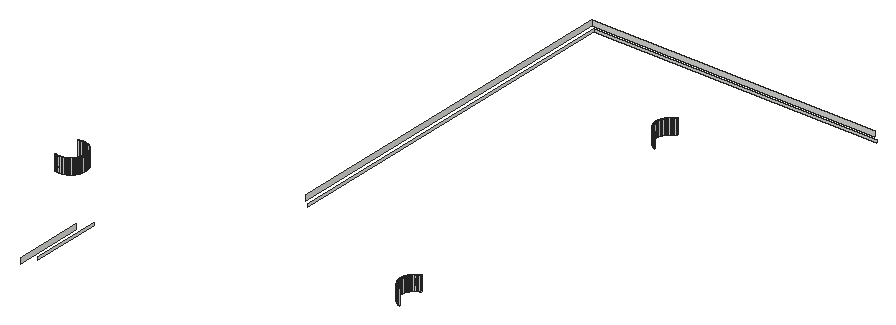
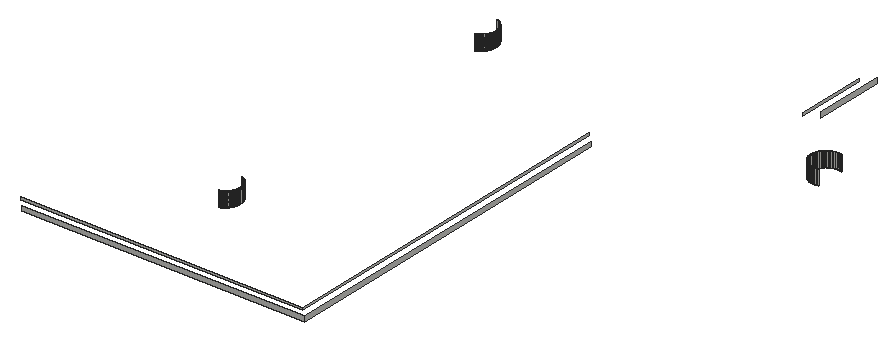
# SketchUp Ruby script. Lengths in inches.
U = 1.inch
M = Sketchup.active_model
def pt(a) = Geom::Point3d.new(a.map { |v| v * U })
def face(e, loops, mat)
  f = e.add_face(loops[0].map { |a| pt(a) })
  loops[1..].each { |l| e.add_face(l.map { |a| pt(a) }).erase! }
  f.material = f.back_material = mat if mat
  f
end
# faces: each face lists its corners as indices into pts; further lists are holes
def faces(e, pts, list, mat = nil) = list.each { |f| face(e, (f[0].is_a?(Array) ? f : [f]).map { |l| l.map { |i| pts[i] } }, mat) }
# xy, xz, yz: faces in a plane at the given z, y or x. An outline is a flat list of corners, or four numbers for a rectangle; further outlines are holes
def ring(l) = l.size == 4 ? [[l[0], l[1]], [l[2], l[1]], [l[2], l[3]], [l[0], l[3]]] : l.each_slice(2).to_a
def flat(e, list, mat, &to3) = list.each { |f| face(e, (f[0].is_a?(Array) ? f : [f]).map { |l| ring(l).map { |u, v| to3.(u, v) } }, mat) }
def xy(e, z, list, mat = nil) = flat(e, list, mat) { |x, y| [x, y, z] }
def xz(e, y, list, mat = nil) = flat(e, list, mat) { |x, z| [x, y, z] }
def yz(e, x, list, mat = nil) = flat(e, list, mat) { |y, z| [x, y, z] }
def lines(e, pts, list) = list.each { |a, b| e.add_line(pt(pts[a]), pt(pts[b])) }
# prism: a flat outline (further loops are holes) pulled along v
def prism(e, loops, v, mat = nil)
  f = face(e, loops, mat); d = Geom::Vector3d.new(v.map { |x| x * U })
  f.pushpull(f.normal.samedirection?(d) ? d.length : -d.length)
end
def box(e, o, s, mat = nil) = prism(e, [[o, [o[0] + s[0], o[1], o[2]], [o[0] + s[0], o[1] + s[1], o[2]], [o[0], o[1] + s[1], o[2]]]], [0, 0, s[2]], mat)
def at(x, y, z, deg = 0) = Geom::Transformation.translation(pt([x, y, z])) * Geom::Transformation.rotation(ORIGIN, Z_AXIS, deg.degrees)
def axes(o, x, y, z) = Geom::Transformation.new([*x, 0, *y, 0, *z, 0, *pt(o).to_a, 1])
def part(name) = M.definitions.add(name)
# library, detail: a bought-in or finely detailed component or shape, given as its bounding box
def library(name, o, s) = part(name).tap { |d| box(d.entities, o, s) }
def detail(e, o, s) = box(e.add_group.entities, o, s)
def put(e, d, t, mat = nil) = e.add_instance(d, t).tap { |i| i.material = mat if mat }
def group(e, t, mat = nil) = e.add_group.tap { |g| g.transformation = t; g.material = mat if mat }.entities
root = M.entities
xz(root,185,[[120.34,108,120.42,111],[120.42,108,120.5,111],[120.5,108,120.58,111],[120.58,108,120.66,111]])
xz(root,191,[[120.34,108,120.42,111],[120.42,108,120.5,111],[120.5,108,120.58,111],[120.58,108,120.66,111]])
xz(root,273,[[158,108,215,108.5]])
xz(root,275,[[156,107.5,213,108.5]])
yz(root,123.5,[[187.84,108,187.92,111],[187.92,108,188,111],[188,108,188.08,111],[188.08,108,188.16,111]])
yz(root,133.5,[[159,107.5,173,108.5]])
yz(root,135.5,[[161,108,175,108.5]])
yz(root,156,[[203,107.5,275,108.5]])
yz(root,158,[[201,108,273,108.5]])
yz(root,187,[[187.84,108,187.92,111],[187.92,108,188,111],[188,108,188.08,111],[188.08,108,188.16,111],[252.34,108,252.42,111],
  [252.42,108,252.5,111],[252.5,108,252.58,111],[252.58,108,252.66,111]])
p = [[120.03,185.04,108],[119.95,185.05,108],[119.95,185.05,111],[120.03,185.04,111],[120.11,185.03,108],[120.11,185.03,111],
  [120.1875,185.02,108],[120.1875,185.02,111],[120.26,185.01,108],[120.26,185.01,111],[120.34,185,108],[120.34,185,111],
  [120.74,185.01,108],[120.66,185,108],[120.66,185,111],[120.74,185.01,111],[120.8125,185.02,108],[120.8125,185.02,111],
  [120.89,185.03,108],[120.89,185.03,111],[120.97,185.04,108],[120.97,185.04,111],[121.05,185.05,108],[121.05,185.05,111],
  [119.65,185.125,108],[119.57,185.15,108],[119.57,185.15,111],[119.65,185.125,111],[119.72,185.1,108],[119.72,185.1,111],
  [119.8,185.08,108],[119.8,185.08,111],[119.875,185.07,108],[119.875,185.07,111],[121.125,185.07,108],[121.125,185.07,111],
  [121.2,185.08,108],[121.2,185.08,111],[121.28,185.1,108],[121.28,185.1,111],[121.35,185.125,108],[121.35,185.125,111],
  [121.43,185.15,108],[121.43,185.15,111],[121.5,185.17,108],[121.5,185.17,111],[189.07,185.15,108],[189,185.17,108],
  [189,185.17,111],[189.07,185.15,111],[121.58,185.2,108],[121.58,185.2,111],[121.65,185.23,108],[121.65,185.23,111],
  [121.72,185.26,108],[121.72,185.26,111],[188.85,185.23,108],[188.78,185.26,108],[188.78,185.26,111],[188.85,185.23,111],
  [188.92,185.2,108],[188.92,185.2,111],[121.79,185.29,108],[121.79,185.29,111],[121.86,185.33,108],[121.86,185.33,111],
  [121.93,185.36,108],[121.93,185.36,111],[188.64,185.33,108],[188.57,185.36,108],[188.57,185.36,111],[188.64,185.33,111],
  [188.71,185.29,108],[188.71,185.29,111],[122,185.4,108],[122,185.4,111],[122.07,185.44,108],[122.07,185.44,111],
  [122.13,185.48,108],[122.13,185.48,111],[188.43,185.44,108],[188.37,185.48,108],[188.37,185.48,111],[188.43,185.44,111],
  [188.5,185.4,108],[188.5,185.4,111],[122.2,185.53,108],[122.2,185.53,111],[122.26,185.57,108],[122.26,185.57,111],
  [188.3,185.53,108],[188.24,185.57,108],[188.24,185.57,111],[188.3,185.53,111],[122.33,185.62,108],[122.33,185.62,111],
  [122.39,185.67,108],[122.39,185.67,111],[188.17,185.62,108],[188.11,185.67,108],[188.11,185.67,111],[188.17,185.62,111],
  [122.45,185.72,108],[122.45,185.72,111],[122.51,185.77,108],[122.51,185.77,111],[188.05,185.72,108],[187.99,185.77,108],
  [187.99,185.77,111],[188.05,185.72,111],[122.57,185.82,108],[122.57,185.82,111],[122.62,185.88,108],[122.62,185.88,111],
  [187.93,185.82,108],[187.88,185.88,108],[187.88,185.88,111],[187.93,185.82,111],[122.68,185.93,108],[122.68,185.93,111],
  [122.73,185.99,108],[122.73,185.99,111],[187.82,185.93,108],[187.77,185.99,108],[187.77,185.99,111],[187.82,185.93,111],
  [122.78,186.05,108],[122.78,186.05,111],[187.72,186.05,108],[187.72,186.05,111],[122.83,186.11,108],[122.83,186.11,111],
  [122.88,186.17,108],[122.88,186.17,111],[187.67,186.11,108],[187.62,186.17,108],[187.62,186.17,111],[187.67,186.11,111],
  [122.93,186.24,108],[122.93,186.24,111],[122.97,186.3,108],[122.97,186.3,111],[187.57,186.24,108],[187.53,186.3,108],
  [187.53,186.3,111],[187.57,186.24,111],[123.02,186.37,108],[123.02,186.37,111],[187.48,186.37,108],[187.48,186.37,111],
  [123.06,186.43,108],[123.06,186.43,111],[123.1,186.5,108],[123.1,186.5,111],[187.44,186.43,108],[187.4,186.5,108],
  [187.4,186.5,111],[187.44,186.43,111],[123.14,186.57,108],[123.14,186.57,111],[187.36,186.57,108],[187.36,186.57,111],
  [123.17,186.64,108],[123.17,186.64,111],[123.21,186.71,108],[123.21,186.71,111],[187.33,186.64,108],[187.29,186.71,108],
  [187.29,186.71,111],[187.33,186.64,111],[123.24,186.78,108],[123.24,186.78,111],[187.26,186.78,108],[187.26,186.78,111],
  [123.27,186.85,108],[123.27,186.85,111],[187.23,186.85,108],[187.23,186.85,111],[123.3,186.92,108],[123.3,186.92,111],
  [123.33,187,108],[123.33,187,111],[187.2,186.92,108],[187.17,187,108],[187.17,187,111],[187.2,186.92,111],
  [123.35,187.07,108],[123.35,187.07,111],[187.15,187.07,108],[187.15,187.07,111],[123.375,187.15,108],[123.375,187.15,111],
  [123.4,187.22,108],[123.4,187.22,111],[187.125,187.15,108],[187.1,187.22,108],[187.1,187.22,111],[187.125,187.15,111],
  [123.42,187.3,108],[123.42,187.3,111],[187.08,187.3,108],[187.08,187.3,111],[123.43,187.375,108],[123.43,187.375,111],
  [187.07,187.375,108],[187.07,187.375,111],[123.45,187.45,108],[123.45,187.45,111],[187.05,187.45,108],[187.05,187.45,111],
  [123.46,187.53,108],[123.46,187.53,111],[123.47,187.61,108],[123.47,187.61,111],[187.04,187.53,108],[187.03,187.61,108],
  [187.03,187.61,111],[187.04,187.53,111],[123.48,187.6875,108],[123.48,187.6875,111],[187.02,187.6875,108],[187.02,187.6875,111],
  [123.49,187.76,108],[123.49,187.76,111],[187.01,187.76,108],[187.01,187.76,111],[123.5,187.84,108],[123.5,187.84,111],
  [187,187.84,108],[187,187.84,111],[123.48,188.3125,108],[123.49,188.24,108],[123.49,188.24,111],[123.48,188.3125,111],
  [123.5,188.16,108],[123.5,188.16,111],[187,188.16,108],[187.01,188.24,108],[187.01,188.24,111],[187,188.16,111],
  [187.02,188.3125,108],[187.02,188.3125,111],[123.47,188.39,108],[123.47,188.39,111],[187.03,188.39,108],[187.03,188.39,111],
  [123.46,188.47,108],[123.46,188.47,111],[187.04,188.47,108],[187.04,188.47,111],[123.43,188.625,108],[123.45,188.55,108],
  [123.45,188.55,111],[123.43,188.625,111],[187.05,188.55,108],[187.05,188.55,111],[187.07,188.625,108],[187.07,188.625,111],
  [123.42,188.7,108],[123.42,188.7,111],[187.08,188.7,108],[187.08,188.7,111],[123.4,188.78,108],[123.4,188.78,111],
  [187.1,188.78,108],[187.1,188.78,111],[123.375,188.85,108],[123.375,188.85,111],[187.125,188.85,108],[187.125,188.85,111],
  [123.33,189,108],[123.35,188.93,108],[123.35,188.93,111],[123.33,189,111],[187.15,188.93,108],[187.15,188.93,111],
  [187.17,189,108],[187.17,189,111],[123.3,189.08,108],[123.3,189.08,111],[187.2,189.08,108],[187.2,189.08,111],
  [123.24,189.22,108],[123.27,189.15,108],[123.27,189.15,111],[123.24,189.22,111],[187.23,189.15,108],[187.23,189.15,111],
  [187.26,189.22,108],[187.26,189.22,111],[123.21,189.29,108],[123.21,189.29,111],[187.29,189.29,108],[187.29,189.29,111],
  [123.17,189.36,108],[123.17,189.36,111],[187.33,189.36,108],[187.33,189.36,111],[123.1,189.5,108],[123.14,189.43,108],
  [123.14,189.43,111],[123.1,189.5,111],[187.36,189.43,108],[187.36,189.43,111],[187.4,189.5,108],[187.4,189.5,111],
  [123.06,189.57,108],[123.06,189.57,111],[187.44,189.57,108],[187.44,189.57,111],[122.97,189.7,108],[123.02,189.63,108],
  [123.02,189.63,111],[122.97,189.7,111],[187.48,189.63,108],[187.48,189.63,111],[187.53,189.7,108],[187.53,189.7,111],
  [122.93,189.76,108],[122.93,189.76,111],[187.57,189.76,108],[187.57,189.76,111],[122.83,189.89,108],[122.88,189.83,108],
  [122.88,189.83,111],[122.83,189.89,111],[187.62,189.83,108],[187.62,189.83,111],[187.67,189.89,108],[187.67,189.89,111],
  [122.73,190.01,108],[122.78,189.95,108],[122.78,189.95,111],[122.73,190.01,111],[187.72,189.95,108],[187.72,189.95,111],
  [187.77,190.01,108],[187.77,190.01,111],[122.68,190.07,108],[122.68,190.07,111],[187.82,190.07,108],[187.82,190.07,111],
  [122.57,190.18,108],[122.62,190.12,108],[122.62,190.12,111],[122.57,190.18,111],[187.88,190.12,108],[187.88,190.12,111],
  [187.93,190.18,108],[187.93,190.18,111],[122.45,190.28,108],[122.51,190.23,108],[122.51,190.23,111],[122.45,190.28,111],
  [187.99,190.23,108],[187.99,190.23,111],[188.05,190.28,108],[188.05,190.28,111],[122.33,190.38,108],[122.39,190.33,108],
  [122.39,190.33,111],[122.33,190.38,111],[188.11,190.33,108],[188.11,190.33,111],[188.17,190.38,108],[188.17,190.38,111],
  [122.2,190.47,108],[122.26,190.43,108],[122.26,190.43,111],[122.2,190.47,111],[188.24,190.43,108],[188.24,190.43,111],
  [188.3,190.47,108],[188.3,190.47,111],[122.07,190.56,108],[122.13,190.52,108],[122.13,190.52,111],[122.07,190.56,111],
  [188.37,190.52,108],[188.37,190.52,111],[188.43,190.56,108],[188.43,190.56,111],[121.86,190.67,108],[121.93,190.64,108],
  [121.93,190.64,111],[121.86,190.67,111],[122,190.6,108],[122,190.6,111],[188.5,190.6,108],[188.5,190.6,111],
  [188.57,190.64,108],[188.57,190.64,111],[188.64,190.67,108],[188.64,190.67,111],[121.65,190.77,108],[121.72,190.74,108],
  [121.72,190.74,111],[121.65,190.77,111],[121.79,190.71,108],[121.79,190.71,111],[188.71,190.71,108],[188.71,190.71,111],
  [188.78,190.74,108],[188.78,190.74,111],[188.85,190.77,108],[188.85,190.77,111],[121.43,190.85,108],[121.5,190.83,108],
  [121.5,190.83,111],[121.43,190.85,111],[121.58,190.8,108],[121.58,190.8,111],[188.92,190.8,108],[188.92,190.8,111],
  [189,190.83,108],[189,190.83,111],[189.07,190.85,108],[189.07,190.85,111],[119.57,190.85,108],[119.65,190.875,108],
  [119.65,190.875,111],[119.57,190.85,111],[119.72,190.9,108],[119.72,190.9,111],[119.8,190.92,108],[119.8,190.92,111],
  [119.875,190.93,108],[119.875,190.93,111],[119.95,190.95,108],[119.95,190.95,111],[120.03,190.96,108],[120.03,190.96,111],
  [120.97,190.96,108],[121.05,190.95,108],[121.05,190.95,111],[120.97,190.96,111],[121.125,190.93,108],[121.125,190.93,111],
  [121.2,190.92,108],[121.2,190.92,111],[121.28,190.9,108],[121.28,190.9,111],[121.35,190.875,108],[121.35,190.875,111],
  [120.11,190.97,108],[120.11,190.97,111],[120.1875,190.98,108],[120.1875,190.98,111],[120.26,190.99,108],[120.26,190.99,111],
  [120.34,191,108],[120.34,191,111],[120.66,191,108],[120.74,190.99,108],[120.74,190.99,111],[120.66,191,111],
  [120.8125,190.98,108],[120.8125,190.98,111],[120.89,190.97,108],[120.89,190.97,111],[189.07,249.65,108],[189,249.67,108],
  [189,249.67,111],[189.07,249.65,111],[188.85,249.73,108],[188.78,249.76,108],[188.78,249.76,111],[188.85,249.73,111],
  [188.92,249.7,108],[188.92,249.7,111],[188.64,249.83,108],[188.57,249.86,108],[188.57,249.86,111],[188.64,249.83,111],
  [188.71,249.79,108],[188.71,249.79,111],[188.43,249.94,108],[188.37,249.98,108],[188.37,249.98,111],[188.43,249.94,111],
  [188.5,249.9,108],[188.5,249.9,111],[188.3,250.03,108],[188.24,250.07,108],[188.24,250.07,111],[188.3,250.03,111],
  [188.17,250.12,108],[188.11,250.17,108],[188.11,250.17,111],[188.17,250.12,111],[188.05,250.22,108],[187.99,250.27,108],
  [187.99,250.27,111],[188.05,250.22,111],[187.93,250.32,108],[187.88,250.38,108],[187.88,250.38,111],[187.93,250.32,111],
  [187.82,250.43,108],[187.77,250.49,108],[187.77,250.49,111],[187.82,250.43,111],[187.72,250.55,108],[187.72,250.55,111],
  [187.67,250.61,108],[187.62,250.67,108],[187.62,250.67,111],[187.67,250.61,111],[187.57,250.74,108],[187.53,250.8,108],
  [187.53,250.8,111],[187.57,250.74,111],[187.48,250.87,108],[187.48,250.87,111],[187.44,250.93,108],[187.4,251,108],
  [187.4,251,111],[187.44,250.93,111],[187.36,251.07,108],[187.36,251.07,111],[187.33,251.14,108],[187.29,251.21,108],
  [187.29,251.21,111],[187.33,251.14,111],[187.26,251.28,108],[187.26,251.28,111],[187.23,251.35,108],[187.23,251.35,111],
  [187.2,251.42,108],[187.17,251.5,108],[187.17,251.5,111],[187.2,251.42,111],[187.15,251.57,108],[187.15,251.57,111],
  [187.125,251.65,108],[187.1,251.72,108],[187.1,251.72,111],[187.125,251.65,111],[187.08,251.8,108],[187.08,251.8,111],
  [187.07,251.875,108],[187.07,251.875,111],[187.05,251.95,108],[187.05,251.95,111],[187.04,252.03,108],[187.03,252.11,108],
  [187.03,252.11,111],[187.04,252.03,111],[187.02,252.1875,108],[187.02,252.1875,111],[187.01,252.26,108],[187.01,252.26,111],
  [187,252.34,108],[187,252.34,111],[187,252.66,108],[187.01,252.74,108],[187.01,252.74,111],[187,252.66,111],
  [187.02,252.8125,108],[187.02,252.8125,111],[187.03,252.89,108],[187.03,252.89,111],[187.04,252.97,108],[187.04,252.97,111],
  [187.05,253.05,108],[187.05,253.05,111],[187.07,253.125,108],[187.07,253.125,111],[187.08,253.2,108],[187.08,253.2,111],
  [187.1,253.28,108],[187.1,253.28,111],[187.125,253.35,108],[187.125,253.35,111],[187.15,253.43,108],[187.15,253.43,111],
  [187.17,253.5,108],[187.17,253.5,111],[187.2,253.58,108],[187.2,253.58,111],[187.23,253.65,108],[187.23,253.65,111],
  [187.26,253.72,108],[187.26,253.72,111],[187.29,253.79,108],[187.29,253.79,111],[187.33,253.86,108],[187.33,253.86,111],
  [187.36,253.93,108],[187.36,253.93,111],[187.4,254,108],[187.4,254,111],[187.44,254.07,108],[187.44,254.07,111],
  [187.48,254.13,108],[187.48,254.13,111],[187.53,254.2,108],[187.53,254.2,111],[187.57,254.26,108],[187.57,254.26,111],
  [187.62,254.33,108],[187.62,254.33,111],[187.67,254.39,108],[187.67,254.39,111],[187.72,254.45,108],[187.72,254.45,111],
  [187.77,254.51,108],[187.77,254.51,111],[187.82,254.57,108],[187.82,254.57,111],[187.88,254.62,108],[187.88,254.62,111],
  [187.93,254.68,108],[187.93,254.68,111],[187.99,254.73,108],[187.99,254.73,111],[188.05,254.78,108],[188.05,254.78,111],
  [188.11,254.83,108],[188.11,254.83,111],[188.17,254.88,108],[188.17,254.88,111],[188.24,254.93,108],[188.24,254.93,111],
  [188.3,254.97,108],[188.3,254.97,111],[188.37,255.02,108],[188.37,255.02,111],[188.43,255.06,108],[188.43,255.06,111],
  [188.5,255.1,108],[188.5,255.1,111],[188.57,255.14,108],[188.57,255.14,111],[188.64,255.17,108],[188.64,255.17,111],
  [188.71,255.21,108],[188.71,255.21,111],[188.78,255.24,108],[188.78,255.24,111],[188.85,255.27,108],[188.85,255.27,111],
  [188.92,255.3,108],[188.92,255.3,111],[189,255.33,108],[189,255.33,111],[189.07,255.35,108],[189.07,255.35,111],
  [189.15,255.375,108],[189.15,255.375,111]]
faces(root,p,[[0,1,2,3],[4,0,3,5],[6,4,5,7],[8,6,7,9],[10,8,9,11],[12,13,14,15],[16,12,15,17],[18,16,17,19],
  [20,18,19,21],[22,20,21,23],[24,25,26,27],[28,24,27,29],[30,28,29,31],[32,30,31,33],[1,32,33,2],[34,22,23,35],
  [36,34,35,37],[38,36,37,39],[40,38,39,41],[42,40,41,43],[44,42,43,45],[46,47,48,49],[50,44,45,51],[52,50,51,53],
  [54,52,53,55],[56,57,58,59],[60,56,59,61],[47,60,61,48],[62,54,55,63],[64,62,63,65],[66,64,65,67],[68,69,70,71],
  [72,68,71,73],[57,72,73,58],[74,66,67,75],[76,74,75,77],[78,76,77,79],[80,81,82,83],[84,80,83,85],[69,84,85,70],
  [86,78,79,87],[88,86,87,89],[90,91,92,93],[81,90,93,82],[94,88,89,95],[96,94,95,97],[98,99,100,101],[91,98,101,92],
  [102,96,97,103],[104,102,103,105],[106,107,108,109],[99,106,109,100],[110,104,105,111],[112,110,111,113],[114,115,116,117],[107,114,117,108],
  [118,112,113,119],[120,118,119,121],[122,123,124,125],[115,122,125,116],[126,120,121,127],[123,128,129,124],[130,126,127,131],[132,130,131,133],
  [134,135,136,137],[128,134,137,129],[138,132,133,139],[140,138,139,141],[142,143,144,145],[135,142,145,136],[146,140,141,147],[143,148,149,144],
  [150,146,147,151],[152,150,151,153],[154,155,156,157],[148,154,157,149],[158,152,153,159],[155,160,161,156],[162,158,159,163],[164,162,163,165],
  [166,167,168,169],[160,166,169,161],[170,164,165,171],[167,172,173,168],[174,170,171,175],[172,176,177,173],[178,174,175,179],[180,178,179,181],
  [182,183,184,185],[176,182,185,177],[186,180,181,187],[183,188,189,184],[190,186,187,191],[192,190,191,193],[194,195,196,197],[188,194,197,189],
  [198,192,193,199],[195,200,201,196],[202,198,199,203],[200,204,205,201],[206,202,203,207],[204,208,209,205],[210,206,207,211],[212,210,211,213],
  [214,215,216,217],[208,214,217,209],[218,212,213,219],[215,220,221,216],[222,218,219,223],[220,224,225,221],[226,222,223,227],[224,228,229,225],
  [230,231,232,233],[231,234,235,232],[236,237,238,239],[237,240,241,238],[242,230,233,243],[240,244,245,241],[246,242,243,247],[244,248,249,245],
  [250,251,252,253],[251,246,247,252],[248,254,255,249],[254,256,257,255],[258,250,253,259],[256,260,261,257],[262,258,259,263],[260,264,265,261],
  [266,262,263,267],[264,268,269,265],[270,271,272,273],[271,266,267,272],[268,274,275,269],[274,276,277,275],[278,270,273,279],[276,280,281,277],
  [282,283,284,285],[283,278,279,284],[280,286,287,281],[286,288,289,287],[290,282,285,291],[288,292,293,289],[294,290,291,295],[292,296,297,293],
  [298,299,300,301],[299,294,295,300],[296,302,303,297],[302,304,305,303],[306,298,301,307],[304,308,309,305],[310,311,312,313],[311,306,307,312],
  [308,314,315,309],[314,316,317,315],[318,310,313,319],[316,320,321,317],[322,323,324,325],[323,318,319,324],[320,326,327,321],[326,328,329,327],
  [330,331,332,333],[331,322,325,332],[328,334,335,329],[334,336,337,335],[338,330,333,339],[336,340,341,337],[342,343,344,345],[343,338,339,344],
  [340,346,347,341],[346,348,349,347],[350,351,352,353],[351,342,345,352],[348,354,355,349],[354,356,357,355],[358,359,360,361],[359,350,353,360],
  [356,362,363,357],[362,364,365,363],[366,367,368,369],[367,358,361,368],[364,370,371,365],[370,372,373,371],[374,375,376,377],[375,366,369,376],
  [372,378,379,373],[378,380,381,379],[382,383,384,385],[383,386,387,384],[386,374,377,387],[380,388,389,381],[388,390,391,389],[390,392,393,391],
  [394,395,396,397],[395,398,399,396],[398,382,385,399],[392,400,401,393],[400,402,403,401],[402,404,405,403],[406,407,408,409],[407,410,411,408],
  [410,394,397,411],[404,412,413,405],[412,414,415,413],[414,416,417,415],[418,419,420,421],[419,422,423,420],[422,424,425,423],[424,426,427,425],
  [426,428,429,427],[428,430,431,429],[432,433,434,435],[433,436,437,434],[436,438,439,437],[438,440,441,439],[440,442,443,441],[442,406,409,443],
  [430,444,445,431],[444,446,447,445],[446,448,449,447],[448,450,451,449],[452,453,454,455],[453,456,457,454],[456,458,459,457],[458,432,435,459],
  [460,461,462,463],[464,465,466,467],[468,464,467,469],[461,468,469,462],[470,471,472,473],[474,470,473,475],[465,474,475,466],[476,477,478,479],
  [480,476,479,481],[471,480,481,472],[482,483,484,485],[477,482,485,478],[486,487,488,489],[483,486,489,484],[490,491,492,493],[487,490,493,488],
  [494,495,496,497],[491,494,497,492],[498,499,500,501],[495,498,501,496],[499,502,503,500],[504,505,506,507],[502,504,507,503],[508,509,510,511],
  [505,508,511,506],[509,512,513,510],[514,515,516,517],[512,514,517,513],[515,518,519,516],[520,521,522,523],[518,520,523,519],[521,524,525,522],
  [524,526,527,525],[528,529,530,531],[526,528,531,527],[529,532,533,530],[534,535,536,537],[532,534,537,533],[535,538,539,536],[538,540,541,539],
  [540,542,543,541],[544,545,546,547],[542,544,547,543],[545,548,549,546],[548,550,551,549],[550,552,553,551],[554,555,556,557],[555,558,559,556],
  [558,560,561,559],[560,562,563,561],[562,564,565,563],[564,566,567,565],[566,568,569,567],[568,570,571,569],[570,572,573,571],[572,574,575,573],
  [574,576,577,575],[576,578,579,577],[578,580,581,579],[580,582,583,581],[582,584,585,583],[584,586,587,585],[586,588,589,587],[588,590,591,589],
  [590,592,593,591],[592,594,595,593],[594,596,597,595],[596,598,599,597],[598,600,601,599],[600,602,603,601],[602,604,605,603],[604,606,607,605],
  [606,608,609,607],[608,610,611,609],[610,612,613,611],[612,614,615,613],[614,616,617,615],[616,618,619,617],[618,620,621,619],[620,622,623,621],
  [622,624,625,623],[624,626,627,625],[626,628,629,627],[628,630,631,629],[630,632,633,631],[632,634,635,633],[634,636,637,635],[636,638,639,637],
  [638,640,641,639],[640,642,643,641],[642,644,645,643],[644,646,647,645],[646,648,649,647]])
